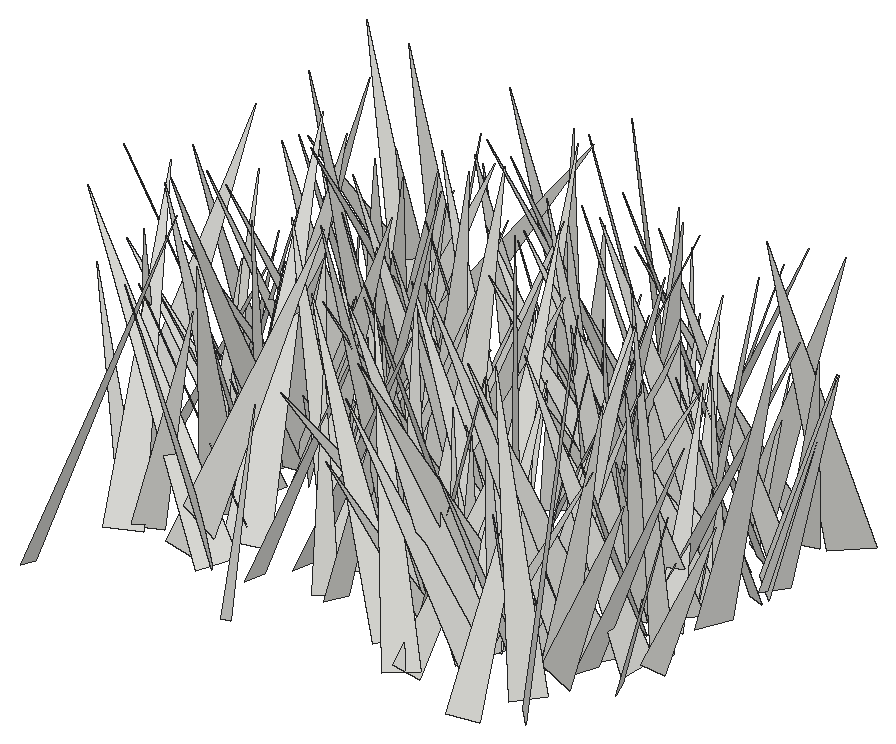
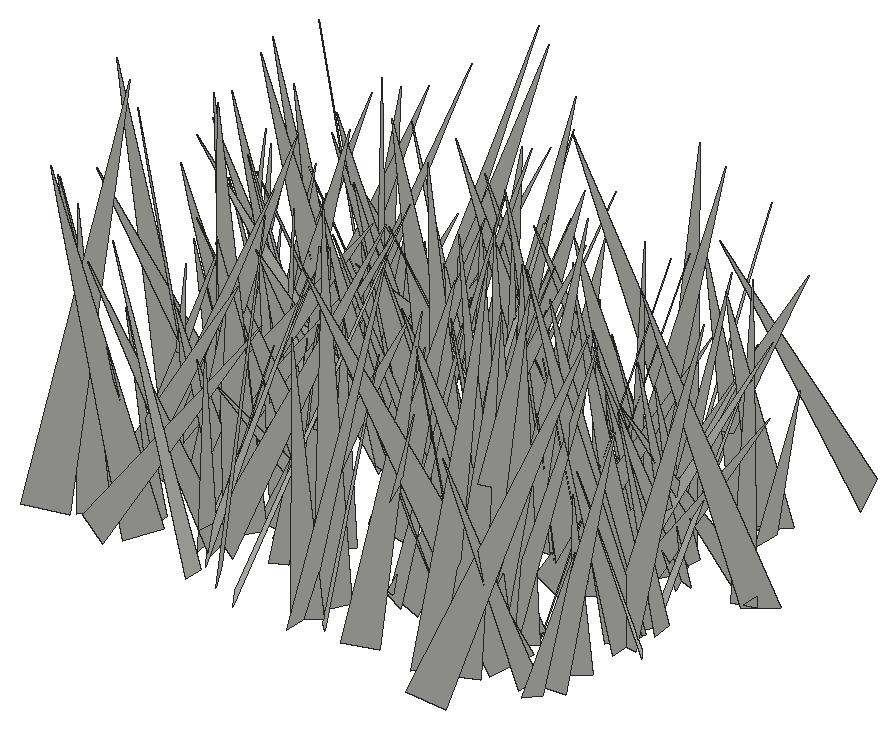
# SketchUp Ruby script. Lengths in inches.
U = 1.inch
M = Sketchup.active_model
def pt(a) = Geom::Point3d.new(a.map { |v| v * U })
def face(e, loops, mat)
  f = e.add_face(loops[0].map { |a| pt(a) })
  loops[1..].each { |l| e.add_face(l.map { |a| pt(a) }).erase! }
  f.material = f.back_material = mat if mat
  f
end
# faces: each face lists its corners as indices into pts; further lists are holes
def faces(e, pts, list, mat = nil) = list.each { |f| face(e, (f[0].is_a?(Array) ? f : [f]).map { |l| l.map { |i| pts[i] } }, mat) }
# xy, xz, yz: faces in a plane at the given z, y or x. An outline is a flat list of corners, or four numbers for a rectangle; further outlines are holes
def ring(l) = l.size == 4 ? [[l[0], l[1]], [l[2], l[1]], [l[2], l[3]], [l[0], l[3]]] : l.each_slice(2).to_a
def flat(e, list, mat, &to3) = list.each { |f| face(e, (f[0].is_a?(Array) ? f : [f]).map { |l| ring(l).map { |u, v| to3.(u, v) } }, mat) }
def xy(e, z, list, mat = nil) = flat(e, list, mat) { |x, y| [x, y, z] }
def xz(e, y, list, mat = nil) = flat(e, list, mat) { |x, z| [x, y, z] }
def yz(e, x, list, mat = nil) = flat(e, list, mat) { |y, z| [x, y, z] }
def lines(e, pts, list) = list.each { |a, b| e.add_line(pt(pts[a]), pt(pts[b])) }
# prism: a flat outline (further loops are holes) pulled along v
def prism(e, loops, v, mat = nil)
  f = face(e, loops, mat); d = Geom::Vector3d.new(v.map { |x| x * U })
  f.pushpull(f.normal.samedirection?(d) ? d.length : -d.length)
end
def box(e, o, s, mat = nil) = prism(e, [[o, [o[0] + s[0], o[1], o[2]], [o[0] + s[0], o[1] + s[1], o[2]], [o[0], o[1] + s[1], o[2]]]], [0, 0, s[2]], mat)
def at(x, y, z, deg = 0) = Geom::Transformation.translation(pt([x, y, z])) * Geom::Transformation.rotation(ORIGIN, Z_AXIS, deg.degrees)
def axes(o, x, y, z) = Geom::Transformation.new([*x, 0, *y, 0, *z, 0, *pt(o).to_a, 1])
def part(name) = M.definitions.add(name)
# library, detail: a bought-in or finely detailed component or shape, given as its bounding box
def library(name, o, s) = part(name).tap { |d| box(d.entities, o, s) }
def detail(e, o, s) = box(e.add_group.entities, o, s)
def put(e, d, t, mat = nil) = e.add_instance(d, t).tap { |i| i.material = mat if mat }
def group(e, t, mat = nil) = e.add_group.tap { |g| g.transformation = t; g.material = mat if mat }.entities
root = M.entities
c1 = part("fur_instance\#9")
p = [[0.8125,0,1.79],[0.67,-0.02,1.48],[0,-0.11,0],[0,0.11,0]]
faces(c1.entities,p,[[0,1,2,3]])
put(root,c1,axes([144.45,341.52,-27.1],[1.52611,3.71718,0.33458],[3.41655,-1.5369,1.49113],[-1.50217,0.28087,3.73135]))
put(root,c1,axes([153.77,344.43,-27.1],[-5.93019,0.58333,0.46706],[0.68124,5.75556,1.46115],[0.30714,-1.50292,5.77689]))
put(root,c1,axes([136.18,340.29,-27.1],[6.68377,2.4417,1.0502],[1.89436,-6.36953,2.75283],[-1.86446,2.28139,6.56175]))
put(root,c1,axes([141.28,344.7,-27.1],[-4.99483,-3.69291,1.05885],[-3.66459,5.10128,0.50484],[1.15306,0.21561,6.19121]))
put(root,c1,axes([153.27,345.17,-27.1],[-6.87965,3.10007,2.46286],[3.78941,6.58637,2.29475],[1.14737,-3.16466,7.18848]))
put(root,c1,axes([156.54,345.66,-27.1],[0.60809,-6.43634,0.77652],[-5.71222,-0.16309,3.1214],[3.06594,0.97271,5.66154]))
put(root,c1,axes([151.9,342.46,-27.1],[-2.77056,6.19265,0.76015],[6.19361,2.62958,1.15202],[-0.75223,-1.15721,6.68563]))
put(root,c1,axes([152.33,348.11,-27.1],[-7.59167,-1.95799,2.55179],[-0.44126,7.11339,4.14535],[3.18601,-3.68034,6.65457]))
put(root,c1,axes([156.14,344.16,-27.1],[-2.17091,-2.72609,1.07786],[-2.90812,2.17161,-0.36485],[0.36901,1.07644,3.46573]))
put(root,c1,axes([149.74,346.48,-27.1],[-4.13984,-2.04423,0.54277],[-1.65039,3.86825,1.98107],[1.32277,-1.57147,4.17043]))
put(root,c1,axes([156.77,343.78,-27.1],[-4.49758,4.50366,1.60112],[4.72062,4.53017,0.51777],[0.74986,-1.50644,6.34374]))
put(root,c1,axes([156.125,344.51,-27.1],[-1.77005,-3.87903,0.89181],[-3.77258,1.32393,-1.7292],[-1.26879,1.475,3.89741]))
put(root,c1,axes([157.48,342.67,-27.1],[5.31201,5.41879,2.20999],[5.24419,-5.73235,1.45032],[-2.59727,-0.49162,7.44831]))
put(root,c1,axes([137.96,345.07,-27.1],[3.51302,-4.23345,1.0034],[-4.35037,-3.40123,0.88101],[0.05668,1.33409,5.43021]))
put(root,c1,axes([155.77,341.2,-27.1],[-5.23053,3.77379,0.03544],[3.44734,4.80229,-2.57973],[1.53577,2.07308,5.91142]))
put(root,c1,axes([150.14,344.08,-27.1],[-3.49983,5.63032,0.78088],[5.54982,3.18646,1.89866],[-1.22869,-1.64469,6.35172]))
put(root,c1,axes([139.46,347.54,-27.1],[4.72004,-5.82808,0.22381],[-5.80637,-4.72269,-0.52693],[-0.55017,-0.15829,7.48115]))
put(root,c1,axes([140.2,344.47,-27.1],[-0.29437,7.39176,2.68978],[7.28817,1.26884,-2.68928],[2.95898,-2.3899,6.89148]))
put(root,c1,axes([141.62,344.51,-27.1],[-4.54084,5.90887,0.08971],[5.53212,4.21055,2.68494],[-2.07809,-1.7025,6.95162]))
put(root,c1,axes([150.23,345.58,-27.1],[5.73054,2.09287,1.0832],[2.24178,-5.71944,-0.8093],[-0.7265,-1.14039,6.04684]))
put(root,c1,axes([146.15,345.19,-27.1],[-2.40866,3.6867,1.3913],[3.88066,2.50239,0.08743],[0.68406,-1.21467,4.40293]))
put(root,c1,axes([143.33,344.62,-27.1],[5.62442,0.34622,0.61815],[0.22701,-5.5658,1.05184],[-0.67115,1.01884,5.53603]))
put(root,c1,axes([153.26,345.5,-27.1],[3.75203,3.55416,0.24846],[3.4305,-3.50645,-1.64561],[0.96201,-1.35805,4.89916]))
put(root,c1,axes([157.1,347.61,-27.1],[2.35436,-6.19743,2.05043],[-5.78585,-2.99044,-2.39512],[-3.02263,0.89697,6.18179]))
put(root,c1,axes([147,349.85,-27.1],[-5.34969,-3.46152,0.37635],[-2.75195,4.62606,3.43064],[2.1332,-2.713,5.36954]))
put(root,c1,axes([156.16,346.19,-27.1],[5.31281,-2.73186,1.51927],[-2.91837,-5.40827,0.48055],[-1.11999,1.13346,5.95467]))
put(root,c1,axes([156,347.41,-27.1],[-8.03194,-0.35365,0.82088],[-0.22203,7.97883,1.26494],[0.86581,-1.23463,7.93959]))
put(root,c1,axes([148.27,347.46,-27.1],[-1.48143,-7.59825,2.03928],[-7.84224,1.26126,-0.99758],[-0.62555,2.18232,7.67677]))
put(root,c1,axes([144.22,346.5,-27.1],[6.32443,-0.86949,0.03215],[-0.87008,-6.31952,0.24926],[0.00213,0.25131,6.37905]))
put(root,c1,axes([136.99,345.31,-27.1],[-4.67353,1.04438,0.03845],[1.02272,4.60667,-0.8165],[0.21505,0.78861,4.71868]))
put(root,c1,axes([153.75,345.71,-27.1],[-4.82421,0.67017,1.12309],[0.52178,4.9221,-0.69578],[1.19925,0.5543,4.82058]))
put(root,c1,axes([152.2,345.31,-27.1],[0.68638,4.30492,0.85677],[4.11958,-0.93113,1.37825],[-1.51508,-0.58153,4.13569]))
put(root,c1,axes([152.04,342.55,-27.1],[-5.06896,3.36354,0.19703],[2.56301,4.08037,-3.71862],[2.18706,3.01393,4.81452]))
put(root,c1,axes([158.91,346.42,-27.1],[3.66327,1.41122,0.72087],[1.44956,-3.71776,-0.08822],[-0.64027,-0.34277,3.92471]))
put(root,c1,axes([137.33,344.43,-27.1],[-3.85678,5.81728,0.33644],[5.7739,3.8696,-0.71896],[0.78484,0.11882,6.94252]))
put(root,c1,axes([158.5,348,-27.1],[-6.51837,1.52305,1.37348],[1.82295,6.39951,1.5551],[0.93967,-1.84981,6.5108]))
put(root,c1,axes([155.05,345.21,-27.1],[-7.31055,-2.64435,2.80127],[-3.45475,7.15889,-2.25809],[1.70424,3.16886,7.43894]))
put(root,c1,axes([140.49,347.61,-27.1],[-3.6362,-3.51378,0.23491],[-3.4583,3.49912,-1.19165],[-0.6648,1.01649,4.91412]))
put(root,c1,axes([157.1,346.75,-27.1],[5.55155,-0.72144,0.45458],[-0.77671,-5.51397,0.73462],[-0.35191,0.78896,5.54982]))
put(root,c1,axes([153.93,346.68,-27.1],[-4.87029,1.64927,0.93909],[1.65484,4.95663,-0.12272],[0.92923,-0.18296,5.1405]))
put(root,c1,axes([150.76,347.75,-27.1],[2.98723,-2.64764,1.00912],[-2.72025,-3.09017,-0.05514],[-0.79284,0.62671,3.99131]))
put(root,c1,axes([150.45,348.66,-27.1],[-3.80657,-5.75041,0.9295],[-5.82495,3.76407,-0.56819],[0.03325,1.08891,6.87272]))
put(root,c1,axes([154.86,347.09,-27.1],[3.44666,-5.98968,2.82803],[-6.61551,-2.95389,1.80641],[0.33028,3.33943,6.67028]))
put(root,c1,axes([146.64,345.24,-27.1],[-7.17026,0.40545,3.85637],[-0.86926,7.73252,-2.42922],[3.77894,2.54801,6.75839]))
put(root,c1,axes([147.41,349.14,-27.1],[4.28198,-1.79299,1.3249],[-1.43721,-4.41332,-1.32759],[-1.70429,-0.78312,4.44833]))
put(root,c1,axes([158.97,348.29,-27.1],[2.19638,-3.75423,0.49776],[-3.62923,-1.92217,1.51658],[1.08198,1.1735,4.07656]))
put(root,c1,axes([147.49,347.82,-27.1],[-3.51582,-2.14374,0.80605],[-2.26912,3.46073,-0.69338],[0.31056,1.01688,4.05904]))
put(root,c1,axes([145.63,346.93,-27.1],[-2.86561,6.0597,1.12131],[6.09085,2.59686,1.53195],[-0.93747,-1.65086,6.5257]))
put(root,c1,axes([134.63,349.51,-27.1],[-0.27546,-6.0552,1.07535],[-6.00995,0.49341,1.23885],[1.30474,0.99438,5.93351]))
put(root,c1,axes([154.86,346.46,-27.1],[3.10305,4.72146,0.30771],[4.72969,-3.10544,-0.04628],[-0.13026,-0.28259,5.64969]))
put(root,c1,axes([146.14,348.77,-27.1],[-0.76363,-5.08076,1.72351],[-5.30047,0.98391,0.55201],[0.83046,1.60796,5.10809]))
put(root,c1,axes([148.84,346.94,-27.1],[-5.6137,1.8249,1.28834],[1.63706,5.7317,-0.98561],[1.51991,0.56669,5.82001]))
put(root,c1,axes([152.98,345.65,-27.1],[-2.31741,7.72302,0.72504],[7.71845,2.37113,-0.58682],[0.77216,-0.52327,8.04183]))
put(root,c1,axes([156.52,350.55,-27.1],[-1.70648,-4.83175,0.15849],[-4.67215,1.69151,1.26205],[1.24174,-0.27565,4.96639]))
put(root,c1,axes([139.04,351.72,-27.1],[0.62863,-8.27068,0.12443],[-8.26435,-0.63324,-0.33804],[-0.34653,0.09834,8.28764]))
put(root,c1,axes([139.91,350.17,-27.1],[2.79879,-2.29313,0.37979],[-2.08936,-2.74248,-1.16161],[-1.01846,-0.6755,3.42672]))
put(root,c1,axes([143.89,347.8125,-27.1],[3.61402,1.40651,0.81578],[1.29809,-3.69316,0.61679],[-0.97915,0.29527,3.8287]))
put(root,c1,axes([145.46,353.45,-27.1],[-5.2335,-6.40482,0.23356],[-5.52847,4.66397,4.0186],[3.24225,-2.38569,7.22925]))
put(root,c1,axes([138.54,349.47,-27.1],[-6.31827,-0.38458,1.65434],[-0.20418,6.49842,0.73085],[1.68614,-0.65417,6.28763]))
put(root,c1,axes([139.84,347.49,-27.1],[4.20978,2.5999,1.29958],[2.36123,-4.39284,1.13935],[-1.69498,0.33775,4.81493]))
put(root,c1,axes([138.58,350.44,-27.1],[-1.9531,-3.93926,0.49775],[-3.87343,2.01224,0.72636],[0.87298,0.11511,4.33645]))
put(root,c1,axes([144.86,349.04,-27.1],[-0.32853,3.96848,1.56907],[4.26678,0.33258,0.05223],[0.07349,-1.56822,3.98171]))
put(root,c1,axes([151.19,349.36,-27.1],[-5.49496,2.98551,0.84144],[3.09795,5.36781,1.18541],[0.15494,-1.44541,6.14025]))
put(root,c1,axes([138.9,350.7,-27.1],[-1.97091,-5.99186,1.73382],[-5.97714,2.33419,1.27215],[1.7839,1.20092,6.17807]))
put(root,c1,axes([141.57,346.31,-27.1],[-2.88963,7.72101,0.14725],[7.7077,2.8933,-0.45358],[0.4764,0.02131,8.23153]))
put(root,c1,axes([149.84,350.59,-27.1],[0.38747,-3.62863,0.53891],[-3.66751,-0.39531,-0.02484],[-0.08219,0.53319,3.64917]))
put(root,c1,axes([138.07,348.48,-27.1],[3.76541,-0.98312,2.37268],[-1.72485,-4.08783,1.04352],[-1.9029,1.75998,3.74912]))
put(root,c1,axes([152.91,347.72,-27.1],[-5.36407,2.31527,0.60969],[2.0889,5.25672,-1.5839],[1.1699,1.22955,5.6236]))
put(root,c1,axes([156.48,350.99,-27.1],[5.03393,-2.19184,1.50174],[-1.99616,-5.24318,-0.96135],[-1.75349,-0.32355,5.40559]))
put(root,c1,axes([141.42,348.4,-27.1],[3.44436,3.22324,0.28553],[3.18394,-3.45028,0.54084],[-0.57733,0.20181,4.68619]))
put(root,c1,axes([153.18,348.375,-27.1],[3.77893,2.89431,1.05154],[2.64296,-3.90266,1.24382],[-1.58036,0.3941,4.59459]))
put(root,c1,axes([147.38,350.33,-27.1],[1.67696,-6.87357,2.26471],[-6.67493,-0.57073,3.21041],[2.79647,2.7596,6.30488]))
put(root,c1,axes([148.54,351.27,-27.1],[-6.39849,-1.36399,1.46981],[-1.16574,6.52941,0.98452],[1.63152,-0.68393,6.46776]))
put(root,c1,axes([136.5,352.24,-27.1],[-3.05725,-3.63504,0.09512],[-3.51202,2.98398,1.15363],[0.94245,-0.67208,4.60753]))
put(root,c1,axes([138.625,350.61,-27.1],[-4.24155,2.82864,0.08548],[2.61337,3.85608,2.07369],[-1.08573,-1.76881,4.65744]))
put(root,c1,axes([155.66,351.67,-27.1],[4.05773,-0.76512,0.97615],[-0.40955,-3.97873,-1.41614],[-1.1707,-1.26007,3.87881]))
put(root,c1,axes([158.76,349.13,-27.1],[-7.01031,-0.43579,1.43561],[-0.72042,6.99511,-1.39453],[1.31601,1.50792,6.88401]))
put(root,c1,axes([148.57,349.02,-27.1],[-4.94866,6.16749,2.69055],[6.18584,5.48419,-1.19385],[2.6481,-1.28527,7.81677]))
put(root,c1,axes([135.56,348.33,-27.1],[4.79921,1.03907,0.41248],[0.79797,-4.45725,1.94381],[-0.78297,1.82633,4.50929]))
put(root,c1,axes([138.25,349.79,-27.1],[-2.58112,4.19595,2.18678],[4.13957,3.20902,-1.27135],[2.29171,-1.07069,4.75939]))
put(root,c1,axes([139.25,350.9,-27.1],[-5.24888,-4.54366,0.15791],[-4.36596,4.97023,-2.11085],[-1.26815,1.69482,6.61361]))
put(root,c1,axes([147.39,350.18,-27.1],[-6.20853,-2.44848,0.56631],[-2.51301,6.03462,-1.45936],[-0.02325,1.56521,6.51238]))
put(root,c1,axes([157.57,352.23,-27.1],[1.87791,-4.76016,0.94457],[-4.63856,-2.05833,-1.15104],[-1.42657,0.4266,4.98606]))
put(root,c1,axes([139.16,352.24,-27.1],[4.92449,-2.5321,0.51516],[-2.43841,-4.92066,-0.87679],[-0.85503,-0.55051,5.46748]))
put(root,c1,axes([141.125,352.88,-27.1],[-0.84326,-5.89202,0.02664],[-5.53518,0.78295,-2.04363],[-2.01949,0.3143,5.59022]))
put(root,c1,axes([145.51,348.45,-27.1],[4.61833,5.37447,0.17353],[5.34108,-4.61135,0.67253],[-0.62281,0.30742,7.05419]))
put(root,c1,axes([134.02,349.29,-27.1],[-1.22058,7.14872,1.6543],[7.02907,1.62036,-1.81584],[2.10547,-1.26529,7.02116]))
put(root,c1,axes([139.85,352.47,-27.1],[2.97269,-7.01093,0.81561],[-6.80259,-2.60982,2.35986],[1.88234,1.64042,7.24024]))
put(root,c1,axes([137.6,349.43,-27.1],[5.0446,1.96996,1.21492],[1.59207,-5.06819,1.60732],[-1.6799,1.1124,5.17158]))
put(root,c1,axes([156.03,350.59,-27.1],[-0.49595,7.7495,2.67586],[7.77568,-0.40515,2.61451],[-2.59882,-2.6911,7.31198]))
put(root,c1,axes([137.68,349.48,-27.1],[0.92539,5.82013,0.73982],[5.78512,-1.02986,0.86568],[-0.97656,-0.58571,5.82931]))
put(root,c1,axes([154.18,347.82,-27.1],[-5.33853,3.8285,0.2094],[3.37353,4.86067,-2.86257],[1.82225,2.21756,5.91295]))
put(root,c1,axes([140.22,351.63,-27.1],[3.37975,2.64749,1.02841],[2.82915,-3.2791,-0.85611],[-0.25046,-1.31446,4.20701]))
put(root,c1,axes([149.52,351.36,-27.1],[-2.08975,2.94897,0.92989],[3.09202,1.98432,0.65582],[-0.0238,-1.13764,3.55435]))
put(root,c1,axes([136.41,353.45,-27.1],[0.97454,-6.53217,0.4424],[-5.83998,-0.6651,3.04417],[2.95966,0.83851,5.86106]))
put(root,c1,axes([152.66,351.77,-27.1],[7.35605,-1.97253,1.00478],[-2.03855,-7.39535,0.40615],[-0.86301,0.65556,7.60509]))
put(root,c1,axes([139.24,354.4,-27.1],[-5.93761,-4.29126,0.84113],[-3.95201,5.87307,2.0655],[1.8719,-1.21235,7.02879]))
put(root,c1,axes([146.56,351.97,-27.1],[5.35038,-4.23141,0.69897],[-4.27634,-5.17862,1.38378],[0.32603,1.51562,6.67957]))
put(root,c1,axes([142.92,351.01,-27.1],[-0.41482,4.98169,1.32883],[5.15587,0.40286,0.09923],[0.00793,-1.33251,4.99795]))
put(root,c1,axes([151.71,349.14,-27.1],[7.40987,3.38689,0.1989],[3.26816,-7.25381,1.76579],[-0.91088,1.52574,7.95356]))
put(root,c1,axes([158.59,352.33,-27.1],[6.87118,-2.4682,1.14103],[-2.53265,-6.93781,0.24398],[-0.98977,0.61792,7.29696]))
put(root,c1,axes([151.6,352.28,-27.1],[5.88028,2.97965,0.94292],[3.11911,-5.72141,-1.37172],[-0.19635,-1.65292,6.44782]))
put(root,c1,axes([152.83,351.8125,-27.1],[3.6305,3.98779,0.322],[3.84064,-3.3521,-1.78874],[1.12055,-1.43096,5.08758]))
put(root,c1,axes([157.6,350.94,-27.1],[-2.09366,4.25191,0.8072],[4.26644,2.17826,-0.40798],[0.72654,-0.53866,4.72184]))
put(root,c1,axes([152.55,354.26,-27.1],[6.00758,0.21792,0.49644],[0.387,-5.59183,-2.22857],[-0.3797,-2.2514,5.58318]))
put(root,c1,axes([138.95,355.93,-27.1],[-5.78164,-4.6449,0.78576],[-4.06196,5.54542,2.89287],[2.386,-1.8147,6.82889]))
put(root,c1,axes([153.2,353.25,-27.1],[-2.5079,-4.6968,1.95628],[-4.90602,2.8103,0.45782],[1.34828,1.48955,5.3047]))
put(root,c1,axes([151.51,354.58,-27.1],[5.83634,-0.86723,1.56304],[-0.35494,-5.79341,-1.88904],[-1.75191,-1.71533,5.58985]))
put(root,c1,axes([154.13,354.67,-27.1],[-6.77007,0.71674,0.61078],[0.8862,6.3486,2.37288],[0.31848,-2.42944,6.38099]))
put(root,c1,axes([144.78,353.69,-27.1],[2.7668,-7.06079,2.0724],[-7.35623,-2.5972,0.97226],[0.18857,2.28135,7.52095]))
put(root,c1,axes([136.3125,354.6,-27.1],[-0.27695,-6.43694,1.01641],[-6.49492,0.18954,-0.56932],[-0.53231,1.03627,6.4177]))
put(root,c1,axes([156.48,353.37,-27.1],[-2.71557,-5.16024,0.69315],[-4.67023,2.06855,-2.89705],[-2.30163,1.89099,5.06058]))
put(root,c1,axes([135.76,352.89,-27.1],[4.33952,0.70183,1.00017],[0.70812,-4.45199,0.05164],[-0.99573,-0.10739,4.3956]))
put(root,c1,axes([156.54,351.4,-27.1],[6.37696,0.70596,0.43543],[0.57496,-6.19552,1.62437],[-0.59783,1.57187,6.20688]))
put(root,c1,axes([150.57,350.04,-27.1],[0.71123,8.26754,0.30404],[8.18462,-0.74766,1.1847],[-1.20692,-0.19821,8.21307]))
put(root,c1,axes([157.59,353.21,-27.1],[-2.51256,7.06983,2.10699],[6.38069,0.96553,4.36915],[-3.70253,-3.13371,6.09968]))
put(root,c1,axes([144.18,352.14,-27.1],[2.59525,5.12132,1.23508],[5.09738,-2.78884,0.85303],[-1.33041,-0.69505,5.67763]))
put(root,c1,axes([141.72,351.77,-27.1],[2.74983,3.97442,1.3241],[3.39736,-3.04242,2.07665],[-2.45097,0.24187,4.36407]))
put(root,c1,axes([145.03,354.15,-27.1],[-6.53044,0.59698,0.86107],[0.69842,6.53195,0.76827],[0.78105,-0.84949,6.51251]))
put(root,c1,axes([151.29,353.11,-27.1],[5.01849,-2.22986,0.6447],[-2.32023,-4.77497,1.54574],[0.06662,1.67347,5.26955]))
put(root,c1,axes([145.6875,352.59,-27.1],[2.61038,6.20008,1.07332],[6.21386,-2.35716,-1.49626],[0.99041,-1.55238,6.55868]))
put(root,c1,axes([151.8,355.7,-27.1],[1.73038,-3.85975,0.19684],[-3.59553,-1.68683,-1.46882],[-1.41726,-0.43309,3.96667]))
put(root,c1,axes([156.68,353.61,-27.1],[-3.91032,-4.73518,3.93684],[-5.20514,5.03349,0.88414],[3.29046,2.33522,6.07707]))
put(root,c1,axes([158.38,353.05,-27.1],[0.93593,4.40998,1.37185],[4.37962,-1.29175,1.16453],[-1.46587,-1.0437,4.3552]))
put(root,c1,axes([158.64,354.71,-27.1],[-2.25031,-4.2676,0.76277],[-4.32128,2.13921,-0.77999],[-0.34742,1.03417,4.76108]))
put(root,c1,axes([141,355.29,-27.1],[-1.51779,-7.89387,2.17922],[-8.18213,1.37007,-0.73587],[-0.33897,2.275,8.00471]))
put(root,c1,axes([156.76,355.51,-27.1],[2.25381,-7.00366,2.80187],[-6.80723,-3.14832,-2.39397],[-3.25014,1.7373,6.957]))
put(root,c1,axes([136.43,354.18,-27.1],[4.89354,-4.52263,1.72188],[-4.82903,-4.72322,1.31813],[-0.31551,2.14541,6.53173]))
put(root,c1,axes([144.41,357.21,-27.1],[-1.51333,-7.7582,0.0595],[-7.60064,1.47034,-1.59746],[-1.5568,0.36304,7.74132]))
put(root,c1,axes([148.1,353.47,-27.1],[-2.07893,6.71015,1.41675],[6.64432,1.60395,2.15305],[-1.69892,-1.93817,6.68674]))
put(root,c1,axes([139.9,356.77,-27.1],[6.8807,-3.2851,0.24825],[-3.20439,-6.80705,-1.26238],[-0.76512,-1.03432,7.51946]))
put(root,c1,axes([148.7,355.35,-27.1],[2.93376,-3.22318,1.07266],[-3.3076,-3.03341,-0.06853],[-0.77414,0.74566,4.35788]))
put(root,c1,axes([153.15,355.78,-27.1],[4.39252,-6.51911,2.0007],[-6.79057,-4.39945,0.57342],[-0.62428,1.98542,7.83991]))
put(root,c1,axes([136.06,354.45,-27.1],[7.69259,-0.4984,1.40276],[-0.64413,-7.77059,0.77146],[-1.3421,0.87272,7.67002]))
put(root,c1,axes([135.27,354.68,-27.1],[2.99336,2.37967,0.42143],[2.41657,-2.95437,-0.48225],[-0.02533,-0.63994,3.79348]))
put(root,c1,axes([152.14,356.76,-27.1],[7.73764,-3.02475,0.93063],[-2.93122,-7.77665,-0.90436],[-1.19293,-0.51074,8.25847]))
put(root,c1,axes([139.2,356.97,-27.1],[5.34448,-4.72432,0.68412],[-4.69665,-5.3877,-0.51471],[-0.85369,0.0645,7.11462]))
put(root,c1,axes([158.33,355.59,-27.1],[3.55889,4.26793,1.49162],[4.48448,-3.09137,-1.85436],[0.57409,-2.30955,5.23854]))
put(root,c1,axes([158.73,355.72,-27.1],[5.12871,-2.48578,0.55768],[-2.53054,-5.11559,0.47007],[-0.29413,0.66743,5.67995]))
put(root,c1,axes([152.27,352.8,-27.1],[3.66299,2.22216,0.32756],[1.7102,-3.16536,2.34915],[-1.4562,1.87225,3.58288]))
put(root,c1,axes([144.73,357.3,-27.1],[-3.08937,-5.14938,0.76665],[-5.09175,3.1744,0.80332],[1.08532,0.23487,5.95105]))
put(root,c1,axes([139.33,357.98,-27.1],[-0.1774,-7.7519,1.13116],[-7.17611,0.61466,3.08685],[3.14245,0.96602,7.113]))
put(root,c1,axes([139.78,356.92,-27.1],[-2.67742,-5.68655,1.10676],[-5.79247,2.6077,-0.61446],[-0.09527,1.2623,6.25523]))
put(root,c1,axes([150.45,356.26,-27.1],[-4.33976,4.07233,1.17149],[4.17045,3.80756,2.21352],[-0.75076,-2.38923,5.52429]))
put(root,c1,axes([149.81,357.72,-27.1],[4.21418,-1.38432,0.79636],[-0.98829,-4.02576,-1.76817],[-1.25452,-1.47878,4.06808]))
put(root,c1,axes([156.38,354.08,-27.1],[-4.08982,2.78235,0.32679],[2.66533,4.04258,-1.06229],[0.86271,0.7007,4.83111]))
put(root,c1,axes([150.1,355.8,-27.1],[-2.43911,-2.15453,1.73505],[-2.51562,2.68975,-0.19638],[1.15067,1.31336,3.24849]))
put(root,c1,axes([151.35,354.68,-27.1],[-1.53438,4.71255,0.03454],[4.47921,1.44703,1.55125],[-1.46492,-0.51147,4.70702]))
put(root,c1,axes([157.04,357.1,-27.1],[-4.74845,-6.02691,1.04144],[-6.05438,4.44477,-1.88271],[-0.8676,1.96887,7.4382]))
put(root,c1,axes([148.62,357.43,-27.1],[0.4786,-6.17329,1.68247],[-6.39725,-0.42884,0.2463],[0.12453,1.69584,6.18692]))
put(root,c1,axes([152.39,357.77,-27.1],[-3.30387,-7.05223,0.96215],[-6.92829,2.9435,-2.21582],[-1.63048,1.78244,7.4659]))
put(root,c1,axes([139.37,356.25,-27.1],[3.36914,-5.54095,2.01408],[-5.73384,-2.5398,2.60427],[1.37175,2.99283,5.93894]))
put(root,c1,axes([143.16,356.54,-27.1],[2.4928,2.63766,0.46244],[2.65596,-2.35455,-0.88721],[0.34203,-0.94022,3.51911]))
put(root,c1,axes([155.22,355.58,-27.1],[-1.00856,5.27208,0.80529],[5.17147,0.76643,1.45913],[-1.30357,-1.0384,5.16556]))
put(root,c1,axes([154.33,354.76,-27.1],[-4.2837,1.86088,0.37109],[1.60299,4.03921,-1.75094],[1.01537,1.47394,4.32979]))
put(root,c1,axes([152.76,357.875,-27.1],[-3.61548,-1.81279,0.7212],[-1.71327,3.67656,0.65243],[0.9333,-0.2734,3.99152]))
put(root,c1,axes([140.04,357.51,-27.1],[0.54062,-3.9189,1.26852],[-4.01221,-0.79056,-0.73238],[-0.93225,1.12979,3.88763]))
put(root,c1,axes([153.51,355.73,-27.1],[-2.74828,4.07366,1.32335],[3.94461,3.01992,-1.10419],[1.66916,-0.42944,4.78838]))
put(root,c1,axes([153.38,357.37,-27.1],[-5.70122,-3.26457,0.62497],[-3.32356,5.6155,-0.98593],[0.04408,1.16649,6.49533]))
put(root,c1,axes([159.01,359.86,-27.1],[4.03591,-7.21522,0.98619],[-7.10178,-4.1491,-1.2924],[-1.61145,0.21471,8.16564]))
put(root,c1,axes([157.43,358.95,-27.1],[2.80299,-5.03768,0.10257],[-5.00094,-2.76705,0.76127],[0.6159,0.45904,5.71449]))
put(root,c1,axes([136.01,357.3,-27.1],[-2.23187,2.81976,1.51549],[3.01775,2.4697,-0.15093],[1.06816,-1.08561,3.59298]))
put(root,c1,axes([141.62,357.09,-27.1],[-4.16616,6.68617,2.08588],[7.00105,3.90518,1.46546],[-0.20279,-2.54114,7.74043]))
put(root,c1,axes([149.46,360.77,-27.1],[-6.65977,-5.09555,0.25994],[-4.96209,6.56797,1.61994],[1.1874,-1.13219,8.22757]))
put(root,c1,axes([136.18,358.85,-27.1],[1.56838,-4.91392,1.31708],[-4.91027,-1.82266,-0.95305],[-1.33063,0.93404,5.06933]))
put(root,c1,axes([155.16,357.94,-27.1],[4.1341,0.32333,0.78637],[0.3951,-4.18703,-0.35553],[-0.75288,-0.42186,4.13146]))
put(root,c1,axes([139.34,360.17,-27.1],[3.47226,-5.91321,0.27335],[-5.89868,-3.48291,-0.41506],[-0.49636,0.02495,6.84473]))
put(root,c1,axes([157.69,357.44,-27.1],[-2.26256,-5.81888,2.33683],[-5.71547,0.89178,-3.31322],[-2.57945,3.12805,5.2916]))
put(root,c1,axes([146.22,359.08,-27.1],[7.26083,-2.43104,1.92439],[-2.31077,-7.51014,-0.76873],[-2.06726,-0.14373,7.61831]))
put(root,c1,axes([140.98,357.64,-27.1],[-3.67972,-3.6806,3.42599],[-4.33109,4.47676,0.15761],[2.55458,2.28831,5.20214]))
put(root,c1,axes([156.18,357.67,-27.1],[1.71748,3.11444,0.84575],[3.20742,-1.75327,-0.057],[-0.35706,-0.7688,3.55615]))
put(root,c1,axes([139.25,362.32,-27.1],[4.10096,-6.21113,0.1393],[-5.64172,-3.79303,-3.03306],[-2.60165,-1.56533,6.79681]))
put(root,c1,axes([138.4375,358.31,-27.1],[5.80573,-6.03364,0.3689],[-5.4436,-4.99608,3.95649],[2.62833,2.98023,7.37953]))
put(root,c1,axes([145.56,360.375,-27.1],[-3.59225,-3.71334,1.0598],[-3.39845,3.72735,1.54069],[1.83374,-0.36648,4.93148]))
put(root,c1,axes([145.77,357.2,-27.1],[-5.65883,0.17912,0.29432],[0.09895,5.4838,-1.43499],[0.33003,1.4272,5.47679]))
put(root,c1,axes([155.01,359.12,-27.1],[6.03076,-3.95506,0.64167],[-4.00583,-5.92637,1.12057],[0.08689,1.28836,7.12438]))
put(root,c1,axes([140.63,360.3,-27.1],[6.98287,-2.99298,2.96369],[-2.61118,-7.57832,-1.50091],[-3.30502,-0.33623,7.44753]))
put(root,c1,axes([143.66,360.625,-27.1],[3.60817,-5.34608,1.25489],[-5.24687,-3.79935,-1.09972],[-1.62036,0.39817,6.35531]))
put(root,c1,axes([152.47,358.6,-27.1],[-6.0406,-4.0795,1.11122],[-4.22494,5.74856,-1.86274],[-0.16426,2.16279,7.04708]))
put(root,c1,axes([156.71,359.9375,-27.1],[-1.84266,-5.86998,0.99209],[-5.21002,1.08759,-3.24178],[-2.88039,1.78795,5.22904]))
put(root,c1,axes([152.29,358.07,-27.1],[6.26365,0.83218,0.34032],[0.77044,-6.2027,0.98722],[-0.46342,0.93576,6.24109]))
put(root,c1,axes([152.79,358.14,-27.1],[-4.924,0.48292,1.1816],[0.20052,4.94285,-1.18453],[1.26062,1.10005,4.80373]))
put(root,c1,axes([150.9,359.82,-27.1],[-6.29622,-3.82649,2.40942],[-4.00808,6.63484,0.06324],[2.09347,1.19444,7.36752]))
put(root,c1,axes([137.07,359.05,-27.1],[4.6922,-0.3007,0.23761],[-0.32477,-4.66947,0.50417],[-0.20347,0.51889,4.67471]))
put(root,c1,axes([146.5,360.7,-27.1],[-7.391,-1.41623,2.02124],[-1.14457,7.62073,1.15434],[2.18657,-0.79801,7.4364]))
put(root,c1,axes([146.41,360.29,-27.1],[2.86346,-4.49186,1.0378],[-4.60706,-2.8331,0.44926],[-0.16992,1.11803,5.30796]))
put(root,c1,axes([151.74,360.29,-27.1],[6.21728,1.67139,0.47713],[1.73743,-6.02723,-1.52629],[-0.05031,-1.59834,6.25448]))
put(root,c1,axes([136.4,359.66,-27.1],[-3.21224,1.96871,0.46482],[2.01704,3.18335,0.45637],[0.15311,-0.63315,3.7398]))
